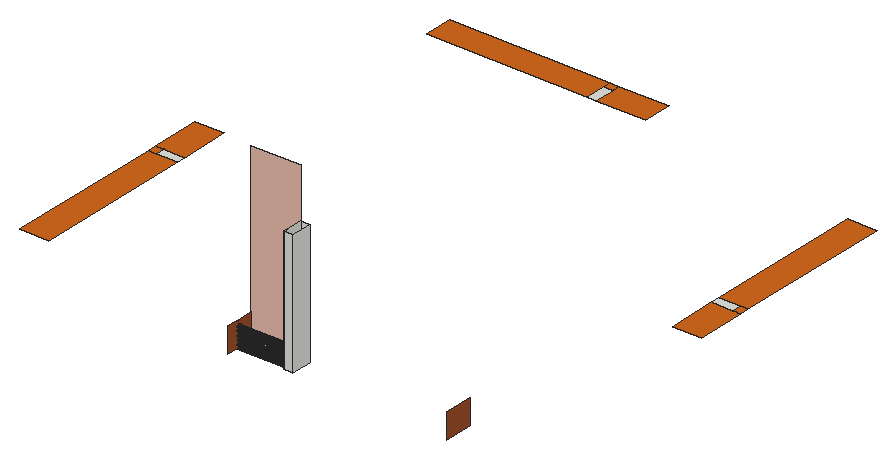
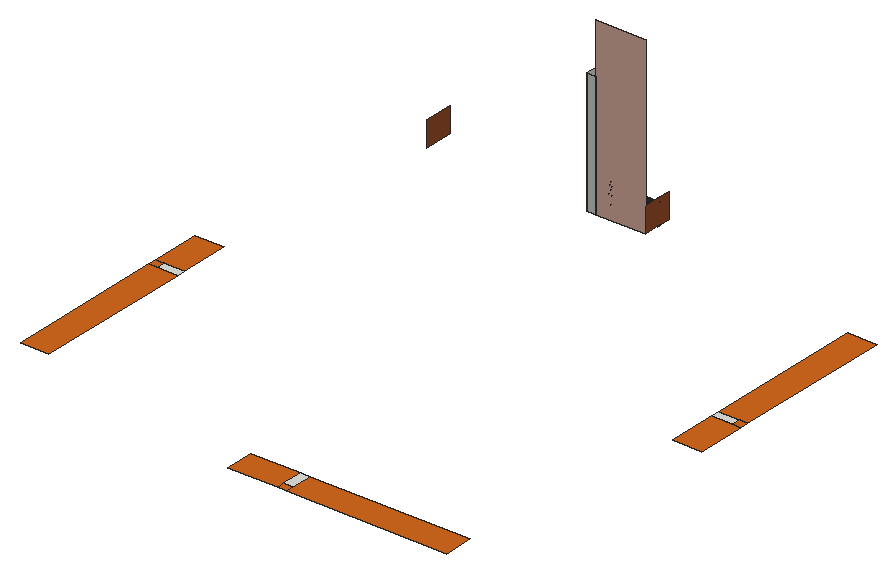
# SketchUp Ruby script. Lengths in inches.
U = 1.inch
M = Sketchup.active_model
def pt(a) = Geom::Point3d.new(a.map { |v| v * U })
def face(e, loops, mat)
  f = e.add_face(loops[0].map { |a| pt(a) })
  loops[1..].each { |l| e.add_face(l.map { |a| pt(a) }).erase! }
  f.material = f.back_material = mat if mat
  f
end
# faces: each face lists its corners as indices into pts; further lists are holes
def faces(e, pts, list, mat = nil) = list.each { |f| face(e, (f[0].is_a?(Array) ? f : [f]).map { |l| l.map { |i| pts[i] } }, mat) }
# xy, xz, yz: faces in a plane at the given z, y or x. An outline is a flat list of corners, or four numbers for a rectangle; further outlines are holes
def ring(l) = l.size == 4 ? [[l[0], l[1]], [l[2], l[1]], [l[2], l[3]], [l[0], l[3]]] : l.each_slice(2).to_a
def flat(e, list, mat, &to3) = list.each { |f| face(e, (f[0].is_a?(Array) ? f : [f]).map { |l| ring(l).map { |u, v| to3.(u, v) } }, mat) }
def xy(e, z, list, mat = nil) = flat(e, list, mat) { |x, y| [x, y, z] }
def xz(e, y, list, mat = nil) = flat(e, list, mat) { |x, z| [x, y, z] }
def yz(e, x, list, mat = nil) = flat(e, list, mat) { |y, z| [x, y, z] }
def lines(e, pts, list) = list.each { |a, b| e.add_line(pt(pts[a]), pt(pts[b])) }
# prism: a flat outline (further loops are holes) pulled along v
def prism(e, loops, v, mat = nil)
  f = face(e, loops, mat); d = Geom::Vector3d.new(v.map { |x| x * U })
  f.pushpull(f.normal.samedirection?(d) ? d.length : -d.length)
end
def box(e, o, s, mat = nil) = prism(e, [[o, [o[0] + s[0], o[1], o[2]], [o[0] + s[0], o[1] + s[1], o[2]], [o[0], o[1] + s[1], o[2]]]], [0, 0, s[2]], mat)
def at(x, y, z, deg = 0) = Geom::Transformation.translation(pt([x, y, z])) * Geom::Transformation.rotation(ORIGIN, Z_AXIS, deg.degrees)
def axes(o, x, y, z) = Geom::Transformation.new([*x, 0, *y, 0, *z, 0, *pt(o).to_a, 1])
def part(name) = M.definitions.add(name)
# library, detail: a bought-in or finely detailed component or shape, given as its bounding box
def library(name, o, s) = part(name).tap { |d| box(d.entities, o, s) }
def detail(e, o, s) = box(e.add_group.entities, o, s)
def put(e, d, t, mat = nil) = e.add_instance(d, t).tap { |i| i.material = mat if mat }
def group(e, t, mat = nil) = e.add_group.tap { |g| g.transformation = t; g.material = mat if mat }.entities
root = M.entities
M.materials.add("[0041_Chocolate]").color = [210, 105, 30]
M.materials.add("[0042_Sienna]").color = [160, 82, 45]
M.materials.add("[0119_RosyBrown]").color = [234, 190, 174]
xy(root,1066.89,[[72,636.29,132,662.8],[1488,886.83,1548,913.33],[671.48,1452.8125,697.99,1512.8125]])
xy(root,1066.89,[[48,169.92,132,636.29],[48,636.29,72,662.8],[48,662.8,132,806.17],[1488,743.45,1572,886.83],[1548,886.83,1572,913.33],
  [1488,913.33,1572,1379.7],[205.11,1452.8125,671.48,1536.8125],[697.99,1452.8125,841.36,1536.8125],[671.48,1512.8125,697.99,1536.8125]],"[0041_Chocolate]")
xz(root,36.8125,[[922.01,1066.89,948.52,1426.89]])
xz(root,96.8125,[[922.01,1066.89,948.52,1426.89]])
xz(root,96.8125,[[778.64,1066.89,922.01,1573.11]],"[0119_RosyBrown]")
yz(root,778.64,[[12.8125,1066.89,44.875,1066.89,45.15,1067.55,45.73,1068.3125,46.5,1068.9,47.38,1069.27,48.34,1069.39,49.29,1069.27,50.18,1068.9,50.95,1068.3125,51.53,1067.55,51.8,1066.89,96.8125,1066.89,96.8125,1140,51.19,1140,51.53,1139.55,51.9,1138.66,52.03,1137.7,51.9,1136.75,51.53,1135.86,50.95,1135.1,50.18,1134.51,49.29,1134.14,48.34,1134.02,47.38,1134.14,46.5,1134.51,45.73,1135.1,45.15,1135.86,44.78,1136.75,44.65,1137.7,44.78,1138.66,45.15,1139.55,45.49,1140,12.8125,1140],[44.875,1066.89,51.8,1066.89,51.53,1067.55,50.95,1068.3125,50.18,1068.9,49.29,1069.27,48.34,1069.39,47.38,1069.27,46.5,1068.9,45.73,1068.3125,45.15,1067.55]],"[0042_Sienna]")
yz(root,922.01,[[[36.8125,1066.89,36.8125,1426.89,44.875,1426.89,44.78,1426.66,44.65,1425.7,44.78,1424.75,45.15,1423.86,45.73,1423.1,46.5,1422.51,47.38,1422.14,48.34,1422.02,49.29,1422.14,50.18,1422.51,50.95,1423.1,51.53,1423.86,51.9,1424.75,52.03,1425.7,51.9,1426.66,51.8,1426.89,96.8125,1426.89,96.8125,1066.89,51.8,1066.89,51.53,1067.55,50.95,1068.3125,50.18,1068.9,49.29,1069.27,48.34,1069.39,47.38,1069.27,46.5,1068.9,45.73,1068.3125,45.15,1067.55,44.875,1066.89],[48.34,1218.02,49.29,1218.14,50.18,1218.51,50.95,1219.1,51.53,1219.86,51.9,1220.75,52.03,1221.7,51.9,1222.66,51.53,1223.55,50.95,1224.3125,50.18,1224.9,49.29,1225.27,48.34,1225.39,47.38,1225.27,46.5,1224.9,45.73,1224.3125,45.15,1223.55,44.78,1222.66,44.65,1221.7,44.78,1220.75,45.15,1219.86,45.73,1219.1,46.5,1218.51,47.38,1218.14]],[44.875,1066.89,45.15,1067.55,45.73,1068.3125,46.5,1068.9,47.38,1069.27,48.34,1069.39,49.29,1069.27,50.18,1068.9,50.95,1068.3125,51.53,1067.55,51.8,1066.89]])
yz(root,948.52,[[36.8125,1066.89,96.8125,1426.89]])
yz(root,1414.89,[[12.8125,1066.89,96.8125,1140]],"[0042_Sienna]")
p = [[922.01,44.65,1065.7],[922.01,44.78,1066.66],[778.64,44.78,1066.66],[778.64,44.65,1065.7],[922.01,51.9,1066.66],[922.01,52.03,1065.7],
  [778.64,52.03,1065.7],[778.64,51.9,1066.66],[922.01,44.875,1066.89],[922.01,45.15,1067.55],[778.64,45.15,1067.55],[778.64,44.875,1066.89],
  [922.01,51.53,1067.55],[922.01,51.8,1066.89],[778.64,51.8,1066.89],[778.64,51.53,1067.55],[922.01,45.73,1068.3125],[778.64,45.73,1068.3125],
  [922.01,50.95,1068.3125],[778.64,50.95,1068.3125],[922.01,46.5,1068.9],[778.64,46.5,1068.9],[922.01,50.18,1068.9],[778.64,50.18,1068.9],
  [922.01,47.38,1069.27],[778.64,47.38,1069.27],[922.01,49.29,1069.27],[778.64,49.29,1069.27],[922.01,48.34,1069.39],[778.64,48.34,1069.39],
  [922.01,48.34,1074.02],[922.01,47.38,1074.14],[778.64,47.38,1074.14],[778.64,48.34,1074.02],[922.01,49.29,1074.14],[778.64,49.29,1074.14],
  [922.01,46.5,1074.51],[778.64,46.5,1074.51],[922.01,50.18,1074.51],[778.64,50.18,1074.51],[922.01,45.73,1075.1],[778.64,45.73,1075.1],
  [922.01,50.95,1075.1],[778.64,50.95,1075.1],[922.01,45.15,1075.86],[778.64,45.15,1075.86],[922.01,51.53,1075.86],[778.64,51.53,1075.86],
  [922.01,44.78,1076.75],[778.64,44.78,1076.75],[922.01,51.9,1076.75],[778.64,51.9,1076.75],[922.01,44.65,1077.7],[778.64,44.65,1077.7],
  [922.01,52.03,1077.7],[778.64,52.03,1077.7],[922.01,44.78,1078.66],[778.64,44.78,1078.66],[922.01,51.9,1078.66],[778.64,51.9,1078.66],
  [922.01,45.15,1079.55],[778.64,45.15,1079.55],[922.01,51.53,1079.55],[778.64,51.53,1079.55],[922.01,45.73,1080.3125],[778.64,45.73,1080.3125],
  [922.01,50.95,1080.3125],[778.64,50.95,1080.3125],[922.01,46.5,1080.9],[778.64,46.5,1080.9],[922.01,50.18,1080.9],[778.64,50.18,1080.9],
  [922.01,47.38,1081.27],[778.64,47.38,1081.27],[922.01,49.29,1081.27],[778.64,49.29,1081.27],[922.01,48.34,1081.39],[778.64,48.34,1081.39],
  [922.01,48.34,1086.02],[922.01,47.38,1086.14],[778.64,47.38,1086.14],[778.64,48.34,1086.02],[922.01,49.29,1086.14],[778.64,49.29,1086.14],
  [922.01,46.5,1086.51],[778.64,46.5,1086.51],[922.01,50.18,1086.51],[778.64,50.18,1086.51],[922.01,45.73,1087.1],[778.64,45.73,1087.1],
  [922.01,50.95,1087.1],[778.64,50.95,1087.1],[922.01,45.15,1087.86],[778.64,45.15,1087.86],[922.01,51.53,1087.86],[778.64,51.53,1087.86],
  [922.01,44.78,1088.75],[778.64,44.78,1088.75],[922.01,51.9,1088.75],[778.64,51.9,1088.75],[922.01,44.65,1089.7],[778.64,44.65,1089.7],
  [922.01,52.03,1089.7],[778.64,52.03,1089.7],[922.01,44.78,1090.66],[778.64,44.78,1090.66],[922.01,51.9,1090.66],[778.64,51.9,1090.66],
  [922.01,45.15,1091.55],[778.64,45.15,1091.55],[922.01,51.53,1091.55],[778.64,51.53,1091.55],[922.01,45.73,1092.3125],[778.64,45.73,1092.3125],
  [922.01,50.95,1092.3125],[778.64,50.95,1092.3125],[922.01,46.5,1092.9],[778.64,46.5,1092.9],[922.01,50.18,1092.9],[778.64,50.18,1092.9],
  [922.01,47.38,1093.27],[778.64,47.38,1093.27],[922.01,49.29,1093.27],[778.64,49.29,1093.27],[922.01,48.34,1093.39],[778.64,48.34,1093.39],
  [922.01,48.34,1098.02],[922.01,47.38,1098.14],[778.64,47.38,1098.14],[778.64,48.34,1098.02],[922.01,49.29,1098.14],[778.64,49.29,1098.14],
  [922.01,46.5,1098.51],[778.64,46.5,1098.51],[922.01,50.18,1098.51],[778.64,50.18,1098.51],[922.01,45.73,1099.1],[778.64,45.73,1099.1],
  [922.01,50.95,1099.1],[778.64,50.95,1099.1],[922.01,45.15,1099.86],[778.64,45.15,1099.86],[922.01,51.53,1099.86],[778.64,51.53,1099.86],
  [922.01,44.78,1100.75],[778.64,44.78,1100.75],[922.01,51.9,1100.75],[778.64,51.9,1100.75],[922.01,44.65,1101.7],[778.64,44.65,1101.7],
  [922.01,52.03,1101.7],[778.64,52.03,1101.7],[922.01,44.78,1102.66],[778.64,44.78,1102.66],[922.01,51.9,1102.66],[778.64,51.9,1102.66],
  [922.01,45.15,1103.55],[778.64,45.15,1103.55],[922.01,51.53,1103.55],[778.64,51.53,1103.55],[922.01,45.73,1104.3125],[778.64,45.73,1104.3125],
  [922.01,50.95,1104.3125],[778.64,50.95,1104.3125],[922.01,46.5,1104.9],[778.64,46.5,1104.9],[922.01,50.18,1104.9],[778.64,50.18,1104.9],
  [922.01,47.38,1105.27],[778.64,47.38,1105.27],[922.01,49.29,1105.27],[778.64,49.29,1105.27],[922.01,48.34,1105.39],[778.64,48.34,1105.39],
  [922.01,48.34,1110.02],[922.01,47.38,1110.14],[778.64,47.38,1110.14],[778.64,48.34,1110.02],[922.01,49.29,1110.14],[778.64,49.29,1110.14],
  [922.01,46.5,1110.51],[778.64,46.5,1110.51],[922.01,50.18,1110.51],[778.64,50.18,1110.51],[922.01,45.73,1111.1],[778.64,45.73,1111.1],
  [922.01,50.95,1111.1],[778.64,50.95,1111.1],[922.01,45.15,1111.86],[778.64,45.15,1111.86],[922.01,51.53,1111.86],[778.64,51.53,1111.86],
  [922.01,44.78,1112.75],[778.64,44.78,1112.75],[922.01,51.9,1112.75],[778.64,51.9,1112.75],[922.01,44.65,1113.7],[778.64,44.65,1113.7],
  [922.01,52.03,1113.7],[778.64,52.03,1113.7],[922.01,44.78,1114.66],[778.64,44.78,1114.66],[922.01,51.9,1114.66],[778.64,51.9,1114.66],
  [922.01,45.15,1115.55],[778.64,45.15,1115.55],[922.01,51.53,1115.55],[778.64,51.53,1115.55],[922.01,45.73,1116.3125],[778.64,45.73,1116.3125],
  [922.01,50.95,1116.3125],[778.64,50.95,1116.3125],[922.01,46.5,1116.9],[778.64,46.5,1116.9],[922.01,50.18,1116.9],[778.64,50.18,1116.9],
  [922.01,47.38,1117.27],[778.64,47.38,1117.27],[922.01,49.29,1117.27],[778.64,49.29,1117.27],[922.01,48.34,1117.39],[778.64,48.34,1117.39],
  [922.01,48.34,1122.02],[922.01,47.38,1122.14],[778.64,47.38,1122.14],[778.64,48.34,1122.02],[922.01,49.29,1122.14],[778.64,49.29,1122.14],
  [922.01,46.5,1122.51],[778.64,46.5,1122.51],[922.01,50.18,1122.51],[778.64,50.18,1122.51],[922.01,45.73,1123.1],[778.64,45.73,1123.1],
  [922.01,50.95,1123.1],[778.64,50.95,1123.1],[922.01,45.15,1123.86],[778.64,45.15,1123.86],[922.01,51.53,1123.86],[778.64,51.53,1123.86],
  [922.01,44.78,1124.75],[778.64,44.78,1124.75],[922.01,51.9,1124.75],[778.64,51.9,1124.75],[922.01,44.65,1125.7],[778.64,44.65,1125.7],
  [922.01,52.03,1125.7],[778.64,52.03,1125.7],[922.01,44.78,1126.66],[778.64,44.78,1126.66],[922.01,51.9,1126.66],[778.64,51.9,1126.66],
  [922.01,45.15,1127.55],[778.64,45.15,1127.55],[922.01,51.53,1127.55],[778.64,51.53,1127.55],[922.01,45.73,1128.3125],[778.64,45.73,1128.3125],
  [922.01,50.95,1128.3125],[778.64,50.95,1128.3125],[922.01,46.5,1128.9],[778.64,46.5,1128.9],[922.01,50.18,1128.9],[778.64,50.18,1128.9],
  [922.01,47.38,1129.27],[778.64,47.38,1129.27],[922.01,49.29,1129.27],[778.64,49.29,1129.27],[922.01,48.34,1129.39],[778.64,48.34,1129.39]]
faces(root,p,[[0,1,2,3],[4,5,6,7],[1,8,9,10,11,2],[12,13,4,7,14,15],[9,16,17,10],[18,12,15,19],[16,20,21,17],[22,18,19,23],
  [20,24,25,21],[26,22,23,27],[24,28,29,25],[28,26,27,29],[30,31,32,33],[34,30,33,35],[31,36,37,32],[38,34,35,39],
  [36,40,41,37],[42,38,39,43],[40,44,45,41],[46,42,43,47],[44,48,49,45],[50,46,47,51],[48,52,53,49],[54,50,51,55],
  [52,56,57,53],[58,54,55,59],[56,60,61,57],[62,58,59,63],[60,64,65,61],[66,62,63,67],[64,68,69,65],[70,66,67,71],
  [68,72,73,69],[74,70,71,75],[72,76,77,73],[76,74,75,77],[78,79,80,81],[82,78,81,83],[79,84,85,80],[86,82,83,87],
  [84,88,89,85],[90,86,87,91],[88,92,93,89],[94,90,91,95],[92,96,97,93],[98,94,95,99],[96,100,101,97],[102,98,99,103],
  [100,104,105,101],[106,102,103,107],[104,108,109,105],[110,106,107,111],[108,112,113,109],[114,110,111,115],[112,116,117,113],[118,114,115,119],
  [116,120,121,117],[122,118,119,123],[120,124,125,121],[124,122,123,125],[126,127,128,129],[130,126,129,131],[127,132,133,128],[134,130,131,135],
  [132,136,137,133],[138,134,135,139],[136,140,141,137],[142,138,139,143],[140,144,145,141],[146,142,143,147],[144,148,149,145],[150,146,147,151],
  [148,152,153,149],[154,150,151,155],[152,156,157,153],[158,154,155,159],[156,160,161,157],[162,158,159,163],[160,164,165,161],[166,162,163,167],
  [164,168,169,165],[170,166,167,171],[168,172,173,169],[172,170,171,173],[174,175,176,177],[178,174,177,179],[175,180,181,176],[182,178,179,183],
  [180,184,185,181],[186,182,183,187],[184,188,189,185],[190,186,187,191],[188,192,193,189],[194,190,191,195],[192,196,197,193],[198,194,195,199],
  [196,200,201,197],[202,198,199,203],[200,204,205,201],[206,202,203,207],[204,208,209,205],[210,206,207,211],[208,212,213,209],[214,210,211,215],
  [212,216,217,213],[218,214,215,219],[216,220,221,217],[220,218,219,221],[222,223,224,225],[226,222,225,227],[223,228,229,224],[230,226,227,231],
  [228,232,233,229],[234,230,231,235],[232,236,237,233],[238,234,235,239],[236,240,241,237],[242,238,239,243],[240,244,245,241],[246,242,243,247],
  [244,248,249,245],[250,246,247,251],[248,252,253,249],[254,250,251,255],[252,256,257,253],[258,254,255,259],[256,260,261,257],[262,258,259,263],
  [260,264,265,261],[266,262,263,267],[264,268,269,265],[268,266,267,269]])
